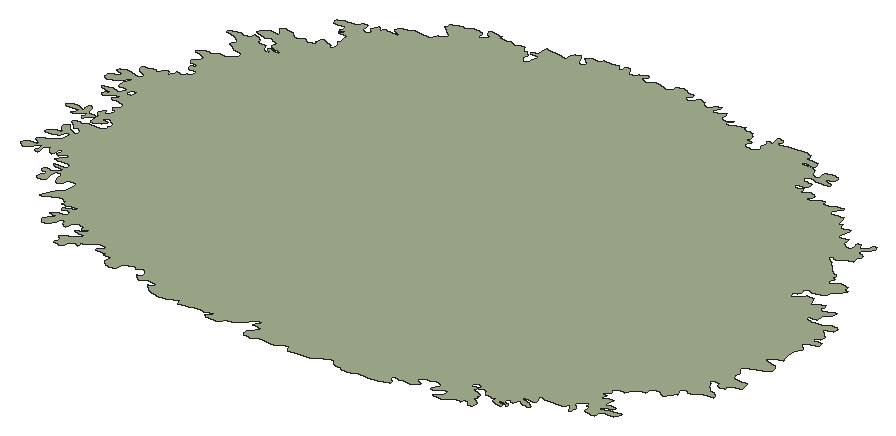
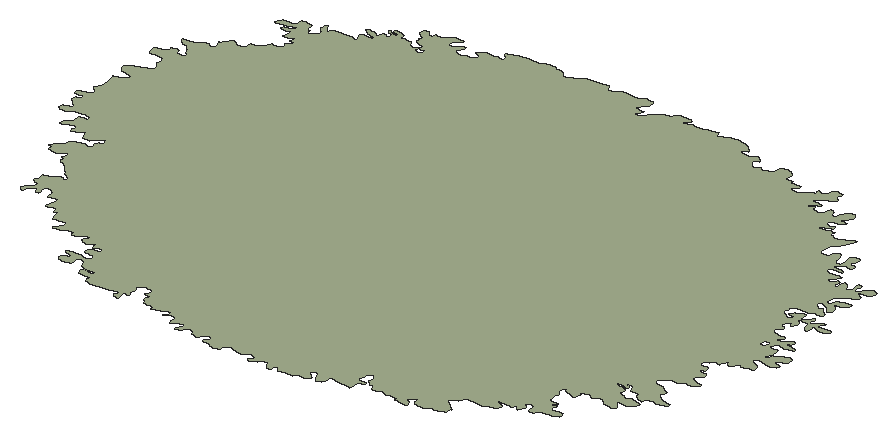
# SketchUp Ruby script. Lengths in inches.
U = 1.inch
M = Sketchup.active_model
def pt(a) = Geom::Point3d.new(a.map { |v| v * U })
def face(e, loops, mat)
  f = e.add_face(loops[0].map { |a| pt(a) })
  loops[1..].each { |l| e.add_face(l.map { |a| pt(a) }).erase! }
  f.material = f.back_material = mat if mat
  f
end
# faces: each face lists its corners as indices into pts; further lists are holes
def faces(e, pts, list, mat = nil) = list.each { |f| face(e, (f[0].is_a?(Array) ? f : [f]).map { |l| l.map { |i| pts[i] } }, mat) }
# xy, xz, yz: faces in a plane at the given z, y or x. An outline is a flat list of corners, or four numbers for a rectangle; further outlines are holes
def ring(l) = l.size == 4 ? [[l[0], l[1]], [l[2], l[1]], [l[2], l[3]], [l[0], l[3]]] : l.each_slice(2).to_a
def flat(e, list, mat, &to3) = list.each { |f| face(e, (f[0].is_a?(Array) ? f : [f]).map { |l| ring(l).map { |u, v| to3.(u, v) } }, mat) }
def xy(e, z, list, mat = nil) = flat(e, list, mat) { |x, y| [x, y, z] }
def xz(e, y, list, mat = nil) = flat(e, list, mat) { |x, z| [x, y, z] }
def yz(e, x, list, mat = nil) = flat(e, list, mat) { |y, z| [x, y, z] }
def lines(e, pts, list) = list.each { |a, b| e.add_line(pt(pts[a]), pt(pts[b])) }
# prism: a flat outline (further loops are holes) pulled along v
def prism(e, loops, v, mat = nil)
  f = face(e, loops, mat); d = Geom::Vector3d.new(v.map { |x| x * U })
  f.pushpull(f.normal.samedirection?(d) ? d.length : -d.length)
end
def box(e, o, s, mat = nil) = prism(e, [[o, [o[0] + s[0], o[1], o[2]], [o[0] + s[0], o[1] + s[1], o[2]], [o[0], o[1] + s[1], o[2]]]], [0, 0, s[2]], mat)
def at(x, y, z, deg = 0) = Geom::Transformation.translation(pt([x, y, z])) * Geom::Transformation.rotation(ORIGIN, Z_AXIS, deg.degrees)
def axes(o, x, y, z) = Geom::Transformation.new([*x, 0, *y, 0, *z, 0, *pt(o).to_a, 1])
def part(name) = M.definitions.add(name)
# library, detail: a bought-in or finely detailed component or shape, given as its bounding box
def library(name, o, s) = part(name).tap { |d| box(d.entities, o, s) }
def detail(e, o, s) = box(e.add_group.entities, o, s)
def put(e, d, t, mat = nil) = e.add_instance(d, t).tap { |i| i.material = mat if mat }
def group(e, t, mat = nil) = e.add_group.tap { |g| g.transformation = t; g.material = mat if mat }.entities
root = M.entities
M.materials.add("Boxwoodplan").color = [166, 177, 144]
xy(root,9.058,[[[125.229,67.129,125.118,67.133,125.023,67.159,124.967,67.215,124.966,67.317,124.992,67.382,125.055,67.445,125.104,67.509,125.163,67.606,124.976,67.635,124.886,67.644,124.906,67.732,124.992,67.79,125.023,67.8,125.018,67.846,124.929,67.877,124.813,67.837,124.716,67.706,124.574,67.551,124.413,67.464,124.307,67.441,124.247,67.416,124.231,67.373,124.086,67.281,123.893,67.251,123.804,67.26,123.723,67.306,123.723,67.328,123.769,67.359,123.859,67.437,123.928,67.483,123.838,67.498,123.726,67.48,123.606,67.436,123.412,67.454,123.315,67.447,123.189,67.403,122.988,67.356,122.899,67.349,122.861,67.443,122.853,67.465,122.786,67.473,122.697,67.454,122.529,67.336,122.329,67.328,122.099,67.353,121.932,67.446,121.79,67.61,121.973,67.702,121.874,67.756,121.738,67.772,121.612,67.749,121.539,67.697,121.459,67.672,121.343,67.738,121.301,67.806,121.388,67.847,121.415,67.907,121.42,67.957,121.379,68.009,121.306,68.085,121.221,68.117,121.134,68.064,121.067,68.038,121.011,68.08,120.995,68.103,120.971,68.121,120.941,68.111,120.862,68.058,120.79,68.01,120.714,67.923,120.703,67.79,120.631,67.749,120.581,67.723,120.521,67.725,120.422,67.746,120.336,67.793,120.292,67.861,120.283,67.951,120.292,68.018,120.305,68.04,120.286,68.08,120.073,68.1,120.141,68.135,120.114,68.136,120.022,68.13,119.852,68.146,119.775,68.173,119.758,68.206,119.772,68.224,119.898,68.314,119.895,68.371,119.811,68.393,119.651,68.39,119.521,68.319,119.423,68.233,119.349,68.199,119.301,68.172,119.3,68.154,119.337,68.101,119.321,68.046,119.25,68.081,119.187,68.121,119.126,68.072,119.103,68.017,119.072,67.904,119.024,67.855,118.951,67.822,118.86,67.816,118.79,67.841,118.772,67.874,118.779,67.892,118.8,67.932,118.822,67.991,118.791,68.048,118.69,68.149,118.804,68.229,118.865,68.269,118.944,68.285,119.012,68.315,119.067,68.37,119.151,68.476,119.08,68.503,119,68.511,118.868,68.53,118.829,68.565,118.837,68.584,118.911,68.62,119.073,68.657,119.116,68.709,119.111,68.748,119.085,68.764,118.935,68.711,118.889,68.732,118.89,68.752,118.912,68.814,118.751,68.825,118.671,68.833,118.617,68.826,118.609,68.806,118.593,68.71,118.578,68.642,118.537,68.591,118.49,68.578,118.47,68.594,118.411,68.639,118.367,68.757,118.327,68.783,118.3,68.784,118.247,68.777,118.24,68.757,118.238,68.641,118.183,68.523,118.123,68.449,118.043,68.419,117.964,68.422,117.917,68.448,117.884,68.506,117.885,68.564,117.938,68.677,118.052,68.784,118.073,68.803,118.059,68.823,118.033,68.829,117.952,68.847,117.872,68.86,117.845,68.875,117.851,68.895,117.872,68.914,118.02,68.982,118.182,69.005,118.224,69.108,118.198,69.169,118.151,69.191,118.123,69.187,117.96,69.168,117.92,69.2,117.926,69.22,117.954,69.279,118.111,69.334,118.283,69.403,118.332,69.442,118.318,69.463,118.222,69.436,118.05,69.417,117.906,69.372,117.817,69.386,117.79,69.392,117.797,69.412,117.817,69.426,117.872,69.47,117.845,69.507,117.817,69.503,117.735,69.511,117.68,69.56,117.666,69.601,117.638,69.597,117.556,69.575,117.399,69.489,117.249,69.413,117.175,69.38,117.12,69.392,117.133,69.412,117.153,69.452,117.179,69.469,117.204,69.55,117.253,69.65,117.285,69.759,117.336,69.812,117.41,69.852,117.454,69.972,117.476,70.112,117.495,70.227,117.491,70.285,117.446,70.321,117.366,70.335,117.279,70.335,117.206,70.31,117.196,70.245,117.196,70.184,117.163,70.124,117.075,70.087,117.019,70.096,116.98,70.155,116.97,70.216,116.944,70.337,116.938,70.4,116.898,70.453,116.87,70.475,116.833,70.491,116.774,70.479,116.739,70.46,116.738,70.428,116.73,70.366,116.732,70.229,116.757,70.167,116.749,70.103,116.699,70.038,116.65,70.01,116.612,69.998,116.575,70.003,116.533,70.011,116.515,70.039,116.511,70.166,116.532,70.223,116.577,70.276,116.593,70.306,116.584,70.334,116.527,70.34,116.446,70.346,116.408,70.362,116.385,70.39,116.382,70.453,116.398,70.483,116.432,70.499,116.605,70.472,116.683,70.497,116.733,70.526,116.793,70.573,116.807,70.636,116.784,70.662,116.74,70.664,116.662,70.67,116.57,70.681,116.469,70.717,116.451,70.746,116.456,70.76,116.476,70.763,116.535,70.775,116.711,70.761,116.8,70.787,116.813,70.844,116.787,70.907,116.715,70.946,116.636,70.953,116.522,70.946,116.423,70.921,116.339,70.939,116.335,70.968,116.356,70.997,116.402,71.054,116.469,71.11,116.522,71.19,116.513,71.224,116.469,71.241,116.404,71.24,116.286,71.14,116.246,71.141,116.212,71.161,116.233,71.22,116.25,71.287,116.206,71.35,116.166,71.366,116.146,71.367,116.141,71.352,116.145,71.306,116.142,71.164,116.101,71.102,116.061,71.108,116.027,71.131,115.929,71.262,115.904,71.327,115.88,71.355,115.864,71.344,115.809,71.293,115.774,71.234,115.793,71.103,115.798,71.037,115.778,70.971,115.729,70.962,115.694,70.978,115.684,71.023,115.704,71.155,115.714,71.233,115.714,71.27,115.699,71.282,115.684,71.272,115.604,71.237,115.565,71.183,115.555,71.12,115.516,71.077,115.379,70.987,115.34,70.977,115.295,70.986,115.216,71.026,115.195,71.056,115.199,71.089,115.232,71.151,115.33,71.237,115.419,71.263,115.509,71.263,115.604,71.267,115.544,71.318,115.392,71.404,115.376,71.466,115.429,71.503,115.52,71.573,115.639,71.635,115.758,71.709,115.793,71.723,115.819,71.746,115.846,71.789,115.849,71.882,115.881,72.003,115.882,72.065,115.861,72.086,115.84,72.095,115.777,72.109,115.743,72.104,115.74,72.088,115.751,71.996,115.71,71.934,115.662,71.899,115.584,71.871,115.513,71.858,115.353,71.833,115.318,71.839,115.304,71.853,115.305,71.86,115.313,71.901,115.33,71.947,115.372,71.995,115.442,72.042,115.5,72.063,115.559,72.065,115.597,72.068,115.617,72.075,115.64,72.096,115.636,72.121,115.581,72.151,115.513,72.207,115.481,72.264,115.477,72.331,115.49,72.382,115.543,72.426,115.569,72.432,115.58,72.425,115.599,72.411,115.642,72.35,115.691,72.304,115.82,72.226,115.893,72.192,115.929,72.177,115.949,72.184,115.973,72.206,115.979,72.222,115.991,72.263,115.975,72.32,115.933,72.366,115.9,72.389,115.867,72.401,115.807,72.401,115.733,72.404,115.689,72.446,115.603,72.519,115.545,72.569,115.506,72.617,115.506,72.646,115.53,72.671,115.587,72.698,115.622,72.703,115.663,72.7,115.723,72.679,115.784,72.677,115.82,72.684,115.855,72.726,115.903,72.757,115.963,72.764,116.034,72.764,116.1875,72.771,116.328,72.792,116.36,72.808,116.361,72.826,116.355,72.868,116.344,72.913,116.355,72.957,116.385,73.06,116.371,73.083,116.349,73.097,116.292,73.126,116.238,73.164,116.166,73.192,116.093,73.195,116.042,73.184,116.021,73.17,115.996,73.119,116.001,73.098,116.013,73.093,116.036,73.088,116.187,73.076,116.213,73.071,116.219,73.0625,116.209,73.046,116.17,73.007,116.124,72.964,116.06,72.928,115.998,72.884,115.925,72.849,115.888,72.852,115.869,72.863,115.843,72.9,115.836,72.995,115.819,73.02,115.837,73.034,115.844,73.077,115.838,73.088,115.826,73.088,115.812,73.087,115.786,73.083,115.753,73.076,115.736,73.065,115.655,72.97,115.623,72.915,115.592,72.892,115.569,72.895,115.543,72.916,115.534,72.932,115.528,72.973,115.556,73.057,115.562,73.102,115.553,73.13,115.532,73.137,115.494,73.128,115.474,73.114,115.428,73.064,115.307,72.957,115.27,72.932,115.245,72.927,115.207,72.935,115.195,72.951,115.287,73.057,115.349,73.102,115.363,73.129,115.363,73.145,115.354,73.152,115.342,73.148,115.328,73.143,115.296,73.131,115.213,73.108,115.045,73.089,114.972,73.096,114.925,73.121,114.903,73.149,114.902,73.165,114.919,73.217,114.966,73.264,115.027,73.281,115.097,73.284,115.172,73.266,115.299,73.223,115.385,73.197,115.397,73.201,115.397,73.209,115.396,73.22,115.387,73.239,115.363,73.287,115.361,73.342,115.369,73.407,115.38,73.437,115.398,73.45,115.446,73.413,115.486,73.363,115.513,73.317,115.522,73.255,115.535,73.204,115.549,73.176,115.573,73.175,115.707,73.157,115.78,73.144,115.815,73.14,115.833,73.154,115.849,73.202,115.793,73.244,115.735,73.309,115.717,73.335,115.717,73.352,115.751,73.46,115.781,73.483,115.809,73.489,115.823,73.477,115.832,73.459,115.861,73.414,115.873,73.39,115.885,73.391,115.906,73.404,115.986,73.482,116.002,73.528,116.004,73.579,115.99,73.611,115.969,73.623,115.905,73.646,115.866,73.666,115.857,73.687,115.873,73.736,115.929,73.773,115.964,73.795,115.977,73.816,115.984,73.869,115.983,73.916,115.887,73.992,115.744,74.014,115.681,74.031,115.647,74.013,115.618,74.014,115.549,74.031,115.53,74.058,115.54,74.082,115.666,74.185,115.659,74.217,115.637,74.233,115.593,74.225,115.564,74.216,115.438,74.154,115.398,74.107,115.348,74.063,115.279,74.049,115.251,74.05,115.204,74.102,115.232,74.126,115.25,74.165,115.282,74.188,115.375,74.22,115.42,74.25,115.41,74.281,115.397,74.283,115.387,74.276,115.361,74.27,115.321,74.273,115.186,74.284,115.04,74.3125,115.016,74.327,115.021,74.347,115.046,74.375,115.259,74.435,115.323,74.434,115.383,74.419,115.444,74.391,115.47,74.393,115.477,74.403,115.526,74.48,115.549,74.495,115.556,74.515,115.555,74.557,115.555,74.583,115.545,74.593,115.531,74.591,115.474,74.591,115.416,74.585,115.369,74.568,115.345,74.576,115.325,74.596,115.3,74.63,115.28,74.718,115.29,74.806,115.32,74.848,115.326,74.88,115.339,74.923,115.377,74.944,115.372,74.99,115.35,75.026,115.261,75.003,115.244,74.969,115.245,74.95,115.248,74.886,115.167,74.839,115.026,74.745,114.871,74.7,114.787,74.725,114.745,74.778,114.735,74.904,114.864,74.99,114.946,75.003,114.99,75.027,115.014,75.061,115.012,75.081,114.927,75.112,114.854,75.138,114.792,75.194,114.827,75.249,114.903,75.278,114.999,75.312,115.064,75.311,115.242,75.267,115.335,75.246,115.419,75.25,115.47,75.269,115.476,75.289,115.461,75.355,115.4,75.407,115.355,75.415,115.243,75.485,115.196,75.527,115.181,75.564,115.175,75.617,115.175,75.644,115.1875,75.659,115.23,75.695,115.281,75.709,115.395,75.741,115.425,75.751,115.466,75.75,115.516,75.746,115.528,75.733,115.543,75.703,115.558,75.689,115.567,75.689,115.596,75.692,115.612,75.704,115.632,75.754,115.66,75.787,115.677,75.81,115.679,75.835,115.696,75.86,115.715,75.872,115.763,75.884,115.802,75.877,115.824,75.833,115.828,75.781,115.844,75.755,115.866,75.754,115.907,75.796,115.932,75.838,115.947,75.942,115.962,75.968,115.995,75.975,116.026,75.974,116.046,75.963,116.067,75.94,116.099,75.94,116.151,75.961,116.196,76.007,116.21,76.032,116.199,76.046,116.259,76.043,116.288,76.046,116.303,76.066,116.308,76.114,116.342,76.155,116.377,76.2,116.323,76.243,116.255,76.272,116.218,76.271,116.186,76.261,116.143,76.249,116.102,76.255,116.08,76.271,116.058,76.295,116.035,76.397,116.048,76.423,116.054,76.439,116.064,76.443,116.168,76.463,116.214,76.472,116.233,76.483,116.223,76.486,116.137,76.514,116.071,76.526,116.043,76.519,116.007,76.52,115.971,76.52,115.936,76.532,115.897,76.582,115.879,76.611,115.879,76.642,115.895,76.663,115.924,76.678,115.955,76.697,115.963,76.725,115.993,76.782,116.02,76.836,116.026,76.89,116.018,76.917,115.978,76.928,115.9,76.954,115.727,77.001,115.692,77.018,115.675,77.042,115.71,77.097,115.755,77.131,115.8,77.159,115.855,77.178,115.908,77.1875,115.96,77.184,116.015,77.16,116.071,77.162,116.097,77.167,116.111,77.187,116.128,77.228,116.165,77.264,116.185,77.282,116.212,77.284,116.281,77.267,116.343,77.256,116.369,77.253,116.393,77.268,116.479,77.336,116.567,77.401,116.62,77.498,116.617,77.542,116.575,77.579,116.458,77.617,116.333,77.647,116.246,77.719,116.189,77.755,116.12,77.776,116.092,77.788,116.079,77.808,116.101,77.855,116.149,77.896,116.147,77.981,116.097,78.06,115.967,78.116,115.727,78.196,115.678,78.212,115.658,78.246,115.729,78.31,115.85,78.362,115.956,78.367,116.013,78.353,116.057,78.327,116.105,78.317,116.158,78.326,116.219,78.337,116.249,78.368,116.263,78.448,116.281,78.483,116.334,78.482,116.391,78.471,116.439,78.451,116.506,78.392,116.531,78.358,116.545,78.318,116.546,78.249,116.552,78.245,116.56,78.249,116.587,78.262,116.639,78.268,116.727,78.271,116.807,78.235,116.842,78.17,116.866,78.092,116.936,78.047,116.977,78.035,116.994,78.034,117.021,78.043,117.117,78.05,117.133,78.055,117.113,78.071,117.05,78.095,116.999,78.099,116.96,78.118,116.941,78.152,116.938,78.164,116.942,78.184,116.957,78.191,116.991,78.192,117.033,78.185,117.14,78.156,117.254,78.152,117.306,78.159,117.325,78.162,117.351,78.173,117.307,78.203,117.265,78.213,117.179,78.228,117.121,78.242,117.081,78.244,117.058,78.248,117.033,78.263,116.982,78.289,116.935,78.315,116.912,78.348,116.923,78.404,116.951,78.442,116.992,78.471,116.952,78.502,116.897,78.517,116.855,78.52,116.799,78.528,116.768,78.555,116.751,78.591,116.736,78.6,116.708,78.599,116.592,78.571,116.54,78.557,116.49,78.559,116.443,78.562,116.393,78.578,116.345,78.595,116.305,78.602,116.219,78.65,116.245,78.662,116.246,78.669,116.258,78.709,116.273,78.745,116.299,78.782,116.33,78.814,116.374,78.839,116.427,78.862,116.473,78.873,116.579,78.867,116.656,78.862,116.689,78.858,116.699,78.857,116.699,78.87,116.691,78.912,116.67,78.956,116.634,78.995,116.592,79.026,116.559,79.073,116.561,79.096,116.571,79.117,116.619,79.147,116.671,79.17,116.697,79.169,116.723,79.163,116.778,79.148,116.845,79.142,116.893,79.127,116.916,79.114,116.935,79.095,116.978,79.055,117.017,79.02,117.062,78.989,117.119,78.976,117.172,78.981,117.218,79.01,117.249,79.046,117.298,79.084,117.324,79.083,117.347,79.069,117.387,79.027,117.434,78.994,117.5625,79.019,117.637,79.037,117.678,79.065,117.684,79.085,117.662,79.102,117.611,79.124,117.602,79.147,117.61,79.169,117.625,79.214,117.632,79.273,117.636,79.299,117.659,79.315,117.687,79.316,117.717,79.308,117.759,79.288,117.893,79.248,117.953,79.226,117.993,79.193,118.019,79.153,118.034,79.13,118.041,79.123,118.051,79.126,118.059,79.131,118.091,79.176,118.097,79.212,118.087,79.315,118.066,79.362,118.042,79.397,118.006,79.436,117.996,79.466,118.008,79.477,118.019,79.475,118.04,79.476,118.04,79.484,118.045,79.508,118.037,79.549,118.023,79.705,118.025,79.782,117.909,79.802,117.812,79.804,117.75,79.8125,117.732,79.819,117.718,79.83,117.731,79.839,117.844,79.882,117.878,79.911,117.878,79.924,117.855,79.948,117.819,79.952,117.766,79.94,117.718,79.918,117.7,79.919,117.685,79.945,117.712,80.028,117.714,80.069,117.714,80.082,117.69,80.103,117.601,80.085,117.488,80.088,117.378,80.105,117.317,80.185,117.315,80.213,117.353,80.25,117.45,80.303,117.498,80.33,117.553,80.335,117.677,80.332,117.769,80.337,117.828,80.346,117.868,80.384,117.909,80.418,117.916,80.461,117.943,80.5,117.998,80.513,118.036,80.509,118.079,80.475,118.09,80.389,118.097,80.3,118.12,80.257,118.176,80.231,118.267,80.212,118.322,80.234,118.34,80.276,118.317,80.319,118.271,80.355,118.214,80.442,118.25,80.521,118.325,80.603,118.344,80.606,118.367,80.576,118.386,80.528,118.461,80.447,118.488,80.421,118.479,80.475,118.461,80.57,118.518,80.587,118.579,80.582,118.706,80.578,118.819,80.575,118.94,80.557,118.959,80.557,118.946,80.587,118.896,80.629,118.765,80.681,118.727,80.689,118.705,80.735,118.707,80.826,118.741,80.871,118.79,80.896,118.906,80.901,119.003,80.91,119.098,80.977,119.225,80.982,119.341,80.971,119.436,80.953,119.557,80.946,119.6,80.991,119.614,81.038,119.657,81.133,119.746,81.187,119.866,81.244,119.877,81.26,119.861,81.294,119.82,81.332,119.713,81.413,119.644,81.487,119.587,81.528,119.53,81.57,119.56,81.577,119.559,81.591,119.555,81.612,119.543,81.679,119.547,81.709,119.582,81.744,119.664,81.785,119.747,81.821,119.786,81.827,119.842,81.826,119.928,81.816,119.952,81.808,119.976,81.81,120.007,81.843,120.059,81.918,120.095,81.932,120.152,81.936,120.254,81.93,120.35,81.898,120.383,81.877,120.412,81.835,120.413,81.765,120.415,81.736,120.42,81.715,120.444,81.704,120.497,81.715,120.542,81.745,120.603,81.798,120.628,81.822,120.65,81.834,120.662,81.85,120.578,81.897,120.54,81.913,120.496,81.956,120.471,82.036,120.472,82.067,120.531,82.083,120.722,82.055,120.819,82.039,120.855,82.026,120.854,81.98,120.864,81.952,120.925,81.948,121.029,81.962,121.13,81.975,121.173,81.971,121.219,81.957,121.247,81.934,121.271,81.933,121.296,81.943,121.44,81.972,121.481,81.981,121.534,81.987,121.57,81.984,121.614,81.957,121.645,81.886,121.671,81.863,121.716,81.844,121.756,81.833,121.796,81.808,121.848,81.753,121.901,81.696,121.888,81.619,121.882,81.545,121.896,81.515,121.927,81.485,121.953,81.461,122,81.453,122.037,81.45,122.081,81.481,122.095,81.512,122.096,81.553,122.084,81.628,122.12,81.787,122.109,81.817,122.091,81.829,122.068,81.833,122.029,81.834,121.977,81.828,121.94,81.826,121.894,81.835,121.868,81.858,121.876,81.88,121.903,81.896,121.943,81.91,121.988,81.937,122.013,82.013,122.016,82.178,122.017,82.21,122.039,82.228,122.066,82.233,122.164,82.222,122.363,82.201,122.455,82.19,122.543,82.169,122.63,82.153,122.681,82.147,122.677,82.355,122.745,82.427,122.829,82.486,122.884,82.477,122.911,82.441,122.96,82.37,122.983,82.297,122.991,82.26,122.989,82.241,123.016,82.206,123.121,82.173,123.173,82.173,123.211,82.204,123.214,82.279,123.112,82.36,123.034,82.419,123.046,82.453,123.09,82.49,123.183,82.541,123.233,82.55,123.314,82.538,123.419,82.537,123.441,82.615,123.651,82.643,123.752,82.661,123.859,82.647,123.939,82.578,123.972,82.543,123.998,82.541,124.038,82.568,124.036,82.643,124.028,82.685,124.04,82.72,124.091,82.729,124.146,82.715,124.217,82.621,124.238,82.548,124.271,82.513,124.319,82.498,124.37,82.503,124.417,82.53,124.505,82.613,124.586,82.668,124.6875,82.715,124.736,82.7,124.749,82.663,124.698,82.592,124.672,82.557,124.68,82.515,124.768,82.457,124.868,82.443,124.919,82.452,124.968,82.498,125.047,82.566,125.161,82.581,125.276,82.553,125.308,82.523,125.384,82.492,125.485,82.511,125.566,82.565,125.566,82.678,125.624,82.721,125.737,82.745,125.842,82.74,125.923,82.681,126.069,82.66,126.122,82.651,126.128,82.614,126.055,82.546,126.022,82.473,126.034,82.437,126.105,82.396,126.208,82.401,126.26,82.433,126.28,82.472,126.301,82.544,126.349,82.567,126.373,82.579,126.425,82.579,126.528,82.541,126.571,82.47,126.656,82.417,126.787,82.447,126.821,82.478,126.828,82.52,126.867,82.603,126.974,82.622,127.004,82.592,127.01,82.55,126.958,82.466,126.909,82.448,126.882,82.413,126.943,82.349,127.073,82.337,127.164,82.373,127.232,82.444,127.256,82.45,127.265,82.433,127.284,82.392,127.308,82.357,127.296,82.301,127.277,82.257,127.295,82.222,127.384,82.179,127.492,82.184,127.547,82.203,127.597,82.258,127.614,82.273,127.617,82.255,127.603,82.212,127.531,82.132,127.497,82.102,127.508,82.066,127.555,82.047,127.612,82.048,127.709,82.088,127.791,82.146,128.011,82.225,128.032,82.153,128.055,82.123,128.107,82.118,128.222,82.11,128.346,82.084,128.361,82.013,128.384,81.983,128.431,81.964,128.454,81.93,128.439,81.892,128.413,81.795,128.529,81.773,128.575,81.755,128.586,81.72,128.512,81.65,128.497,81.613,128.514,81.579,128.589,81.527,128.693,81.5,128.794,81.496,128.906,81.563,128.948,81.639,128.89,81.71,128.857,81.779,128.877,81.885,128.886,81.922,128.857,81.956,128.853,81.992,128.894,82.018,128.995,82.022,128.984,82.122,128.943,82.274,128.992,82.287,129.057,82.275,129.11,82.256,129.142,82.199,129.092,82.131,129.095,82.095,129.142,82.076,129.25,82.076,129.379,82.111,129.887,82.178,129.932,82.168,129.978,82.145,130.025,82.121,130.059,82.097,130.09,82.027,130.072,81.935,130.277,81.949,130.342,81.943,130.426,81.911,130.463,81.805,130.449,81.757,130.432,81.724,130.391,81.717,130.222,81.749,130.157,81.755,130.115,81.755,130.094,81.749,130.091,81.733,130.12,81.685,130.16,81.666,130.208,81.666,130.38,81.681,130.449,81.683,130.534,81.648,130.571,81.609,130.601,81.546,130.669,81.437,130.749,81.398,130.833,81.394,130.864,81.435,130.858,81.518,130.84,81.571,130.847,81.637,130.888,81.687,130.99,81.719,131.099,81.732,131.1875,81.701,131.235,81.659,131.269,81.597,131.27,81.551,131.209,81.495,131.142,81.482,131.101,81.471,131.069,81.437,131.073,81.407,131.123,81.389,131.221,81.363,131.292,81.339,131.312,81.306,131.3,81.275,131.246,81.247,131.158,81.24,130.997,81.233,130.909,81.222,130.821,81.256,130.756,81.269,130.675,81.251,130.618,81.208,130.617,81.143,130.675,81.103,130.762,81.081,130.847,81.066,130.894,81.066,130.928,81.046,130.95,81.003,130.933,80.938,130.898,80.89,130.87,80.866,130.825,80.854,130.682,80.834,130.662,80.829,130.653,80.784,130.658,80.751,130.702,80.732,130.77,80.731,130.811,80.731,130.861,80.746,130.924,80.778,130.938,80.712,130.908,80.665,130.902,80.635,130.941,80.617,131.002,80.622,131.083,80.67,131.139,80.711,131.167,80.736,131.205,80.721,131.269,80.704,131.338,80.651,131.334,80.603,131.291,80.537,131.258,80.472,131.277,80.448,131.324,80.445,131.399,80.456,131.481,80.495,131.52,80.554,131.592,80.597,131.652,80.609,131.689,80.601,131.708,80.577,131.711,80.548,131.694,80.521,131.666,80.497,131.668,80.483,131.688,80.481,131.86,80.499,131.941,80.51,132.008,80.552,132.05,80.589,132.129,80.614,132.226,80.619,132.25,80.595,132.253,80.566,132.092,80.349,132.107,80.304,132.164,80.251,132.247,80.237,132.337,80.255,132.405,80.283,132.489,80.305,132.554,80.213,132.591,79.999,132.592,79.985,132.629,79.974,132.712,79.996,132.723,79.918,132.747,79.871,132.823,79.861,132.961,79.896,133.029,79.893,133.043,79.839,132.975,79.619,132.965,79.567,132.988,79.514,133.054,79.486,133.122,79.496,133.258,79.523,133.278,79.419,133.273,79.316,133.395,79.247,133.527,79.216,133.558,79.318,133.547,79.421,133.525,79.474,133.553,79.525,133.621,79.535,133.66,79.482,133.682,79.429,133.73,79.395,133.808,79.418,133.861,79.467,133.886,79.583,133.889,79.636,133.95,79.659,134.008,79.631,134.038,79.577,134.012,79.455,133.897,79.375,133.844,79.339,133.824,79.282,133.804,79.231,133.826,79.186,133.958,79.161,134.015,79.134,134.019,79.083,133.947,78.997,133.981,78.895,134.011,78.844,133.999,78.794,133.865,78.768,133.763,78.729,133.66,78.658,133.608,78.623,133.543,78.626,133.479,78.659,133.446,78.667,133.42,78.643,133.465,78.549,133.584,78.483,133.63,78.445,133.627,78.396,133.712,78.32,133.879,78.132,134.01,78.05,134.074,78.035,134.111,77.992,134.096,77.898,134.211,77.834,134.148,77.749,134.128,77.697,134.127,77.673,134.158,77.661,134.295,77.679,134.43,77.755,134.559,77.768,134.684,77.734,134.688,77.687,134.621,77.66,134.596,77.644,134.61,77.62,134.6875,77.599,134.759,77.596,134.791,77.595,134.805,77.571,134.716,77.482,134.55,77.322,134.526,77.232,134.522,77.187,134.495,77.142,134.401,77.067,134.273,77.038,134.148,77.043,134.04,77.082,133.97,77.076,133.943,77.004,133.971,76.894,133.941,76.787,133.823,76.72,133.851,76.62,133.989,76.642,134.161,76.833,134.389,76.815,134.465,76.605,134.51,76.595,134.591,76.618,134.679,76.723,134.817,76.735,134.854,76.635,134.804,76.574,134.79,76.539,134.866,76.501,135.005,76.531,135.125,76.598,135.172,76.614,135.261,76.592,135.239,76.477,135.129,76.384,135.064,76.289,135.071,76.113,135.057,76.078,134.965,76.056,134.832,76.087,134.857,75.981,134.989,75.941,135.135,75.936,135.283,75.965,135.52,76.087,135.657,76.099,135.749,76.008,135.716,75.905,135.576,75.849,135.528,75.825,135.5,75.766,135.603,75.675,135.754,75.515,135.722,75.414,135.605,75.359,135.569,75.335,135.608,75.274,135.751,75.269,135.882,75.247,135.893,75.145,135.821,75.089,135.687,75.078,135.562,75.041,135.519,74.942,135.6875,74.761,135.58,74.568,135.584,74.388,135.638,74.176,135.682,74.078,135.549,74.051,135.426,74.008,135.333,73.931,135.305,73.869,135.417,73.801,135.668,73.744,135.745,73.662,135.766,73.559,135.724,73.467,135.61,73.394,135.149,73.234,135.15,73.141,135.194,73.048,135.248,72.954,135.25,72.863,135.241,72.773,135.267,72.719,135.388,72.676,135.513,72.672,135.64,72.682,135.681,72.68,135.739,72.633,135.75,72.453,135.723,72.395,135.614,72.347,135.488,72.33,135.447,72.331,135.4,72.281,135.443,72.191,135.429,72.163,135.345,72.144,135.304,72.145,135.234,72.17,135.201,72.26,135.132,72.292,135.008,72.297,134.966,72.291,134.951,72.233,135.026,72.156,135.113,71.992,135.142,71.969,135.168,71.918,135.185,71.888,135.266,71.877,135.347,71.86,135.432,71.792,135.495,71.71,135.492,71.681,135.407,71.656,135.159,71.616,134.963,71.488,134.89,71.469,134.796,71.544,134.756,71.553,134.692,71.52,134.695,71.435,134.751,71.27,134.709,71.264,134.675,71.219,134.626,71.18,134.573,71.066,134.534,71.019,134.499,71,134.464,71.013,134.341,71.1,134.279,71.115,134.236,71.116,134.191,71.098,134.128,71.063,134.098,70.991,134.107,70.938,134.089,70.874,133.928,70.852,133.875,70.81,133.843,70.759,133.797,70.718,133.785,70.655,133.754,70.609,133.72,70.583,133.682,70.573,133.613,70.564,133.515,70.575,133.455,70.55,133.394,70.502,133.364,70.457,133.438,70.419,133.465,70.376,133.429,70.32,133.375,70.284,133.354,70.225,133.353,70.209,133.351,70.194,133.371,70.186,133.442,70.18,133.468,70.182,133.488,70.182,133.492,70.166,133.455,70.097,133.435,70.049,133.432,70.02,133.473,70.018,133.613,70.094,133.681,70.11,133.763,70.107,133.746,70.004,133.729,69.89,133.729,69.843,133.752,69.82,133.792,69.818,133.855,69.845,133.936,69.846,133.995,69.832,134.035,69.827,134.042,69.798,134.002,69.76,133.923,69.73,133.856,69.722,133.773,69.696,133.734,69.658,133.718,69.602,133.721,69.587,133.761,69.586,133.844,69.611,134.001,69.673,134.156,69.703,134.281,69.705,134.334,69.685,134.309,69.611,134.288,69.569,134.226,69.518,134.074,69.492,133.934,69.491,133.874,69.482,133.843,69.427,133.868,69.308,133.853,69.264,133.772,69.243,133.636,69.255,133.578,69.261,133.534,69.314,133.526,69.426,133.525,69.468,133.513,69.496,133.505,69.511,133.485,69.512,133.426,69.525,133.422,69.581,133.423,69.595,133.42,69.61,133.4,69.614,133.321,69.617,133.263,69.591,133.219,69.536,133.181,69.499,133.157,69.44,133.167,69.391,133.223,69.354,133.298,69.254,133.294,69.155,133.286,69.115,133.278,69.088,133.247,69.066,133.228,69.067,133.206,69.098,133.177,69.157,133.112,69.258,133.071,69.298,133.058,69.312,133.047,69.299,133.04,69.271,133.037,69.227,133.018,69.173,133.012,69.16,132.982,69.144,132.898,69.137,132.758,69.139,132.471,69.14,132.414,69.162,132.327,69.173,132.307,69.163,132.301,69.133,132.352,69.074,132.377,68.976,132.37,68.936,132.339,68.896,132.314,68.889,132.254,68.88,132.151,68.88,132.054,68.884,132.005,68.853,132.061,68.829,132.162,68.814,132.269,68.78,132.344,68.726,132.425,68.654,132.407,68.629,132.347,68.614,132.246,68.621,132.208,68.63,132.158,68.65,132.109,68.684,132.059,68.708,132.024,68.63,132.015,68.558,131.974,68.545,131.918,68.558,131.874,68.589,131.861,68.6,131.842,68.608,131.831,68.59,131.797,68.513,131.798,68.485,131.832,68.448,131.924,68.416,131.962,68.383,131.976,68.34,131.974,68.326,131.954,68.323,131.912,68.36,131.832,68.409,131.738,68.427,131.681,68.429,131.67,68.415,131.691,68.39,131.805,68.347,131.841,68.335,131.865,68.292,131.861,68.264,131.859,68.251,131.816,68.249,131.704,68.26,131.599,68.295,131.564,68.325,131.555,68.371,131.553,68.441,131.503,68.461,131.443,68.442,131.343,68.449,131.245,68.467,131.218,68.489,131.193,68.526,131.197,68.568,131.203,68.583,131.165,68.591,131.071,68.616,131.032,68.618,131.013,68.619,130.978,68.606,130.966,68.577,130.947,68.571,130.92,68.597,130.916,68.612,130.947,68.635,130.962,68.646,130.955,68.671,130.867,68.729,130.83,68.752,130.811,68.756,130.731,68.716,130.711,68.71,130.699,68.681,130.722,68.59,130.818,68.587,130.856,68.582,130.887,68.541,130.88,68.513,130.874,68.499,130.881,68.471,130.993,68.434,131.08,68.396,131.142,68.338,131.158,68.3125,131.157,68.299,131.123,68.283,131.103,68.273,131.134,68.251,131.188,68.225,131.2,68.2,131.15,68.168,131.138,68.141,131.163,68.106,131.248,68.062,131.325,67.994,131.325,67.851,131.303,67.825,131.251,67.814,131.197,67.829,131.16,67.874,131.119,67.939,131.102,67.949,131.064,67.944,131.011,67.926,130.99,67.897,130.991,67.854,130.99,67.84,130.956,67.828,130.78,67.819,130.771,67.826,130.724,67.808,130.68,67.777,130.596,67.692,130.543,67.661,130.47,67.651,130.332,67.643,130.278,67.658,130.275,67.698,130.384,67.762,130.485,67.834,130.482,67.937,130.475,67.98,130.476,67.994,130.444,68.015,130.385,68.034,130.31,68.034,130.227,67.95,130.207,67.911,130.149,67.866,130.135,67.857,130.098,67.865,130.062,67.88,130.049,67.907,130.09,67.999,130.149,68.094,130.151,68.135,130.083,68.189,129.971,68.224,129.92,68.246,129.882,68.238,129.858,68.215,129.824,68.171,129.791,68.156,129.749,68.157,129.693,68.166,129.655,68.168,129.617,68.145,129.537,68.05,129.55,68.01,129.624,67.97,129.679,67.938,129.707,67.917,129.716,67.89,129.692,67.851,129.631,67.807,129.53,67.756,129.474,67.735,129.401,67.738,129.346,67.76,129.273,67.769,129.227,67.745,129.191,67.743,129.159,67.76,129.104,67.766,129.031,67.752,129.008,67.717,129.019,67.659,129.115,67.575,129.143,67.536,129.143,67.497,129.125,67.492,128.836,67.391,128.56,67.369,128.327,67.373,128.237,67.371,128.114,67.31,128.011,67.275,127.914,67.279,127.877,67.281,127.827,67.299,127.779,67.328,127.719,67.325,127.63,67.334,127.546,67.376,127.486,67.433,127.454,67.478,127.396,67.491,127.296,67.479,127.201,67.438,127.12,67.398,127.021,67.325,126.924,67.269,126.831,67.24,126.59,67.222,126.4,67.186,126.304,67.19,126.239,67.284,126.208,67.351,126.119,67.365,126.028,67.352,125.932,67.28,125.867,67.217,125.777,67.21,125.601,67.233,125.415,67.24,125.337,67.189],[115.737,74.415,115.78,74.419,115.799,74.422,115.825,74.431,115.837,74.474,115.838,74.513,115.845,74.597,115.837,74.631,115.825,74.643,115.826,74.658,115.782,74.635,115.726,74.612,115.707,74.606,115.691,74.59,115.669,74.557,115.66,74.52,115.662,74.476,115.681,74.437,115.699,74.421]]],"Boxwoodplan")
